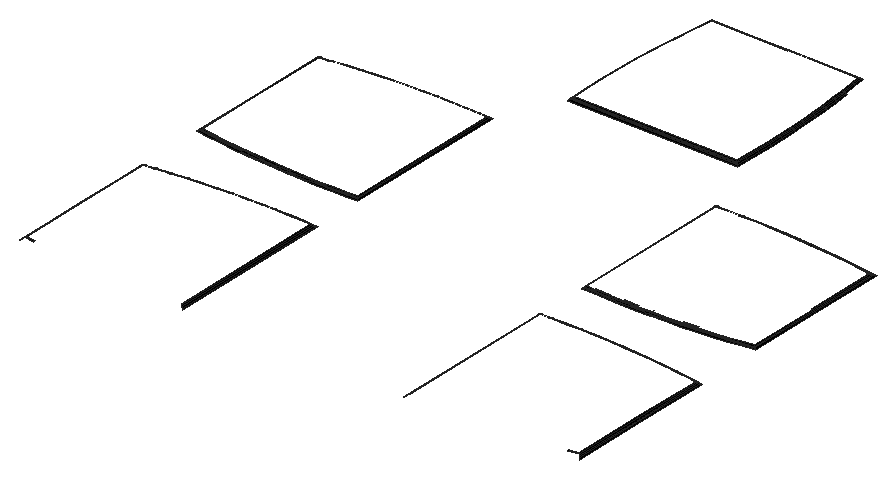
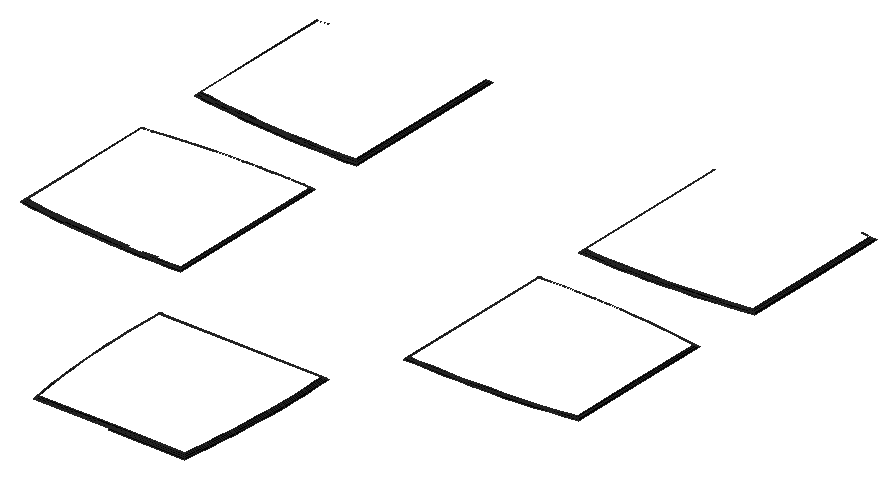
# SketchUp Ruby script. Lengths in inches.
U = 1.inch
M = Sketchup.active_model
def pt(a) = Geom::Point3d.new(a.map { |v| v * U })
def face(e, loops, mat)
  f = e.add_face(loops[0].map { |a| pt(a) })
  loops[1..].each { |l| e.add_face(l.map { |a| pt(a) }).erase! }
  f.material = f.back_material = mat if mat
  f
end
# faces: each face lists its corners as indices into pts; further lists are holes
def faces(e, pts, list, mat = nil) = list.each { |f| face(e, (f[0].is_a?(Array) ? f : [f]).map { |l| l.map { |i| pts[i] } }, mat) }
# xy, xz, yz: faces in a plane at the given z, y or x. An outline is a flat list of corners, or four numbers for a rectangle; further outlines are holes
def ring(l) = l.size == 4 ? [[l[0], l[1]], [l[2], l[1]], [l[2], l[3]], [l[0], l[3]]] : l.each_slice(2).to_a
def flat(e, list, mat, &to3) = list.each { |f| face(e, (f[0].is_a?(Array) ? f : [f]).map { |l| ring(l).map { |u, v| to3.(u, v) } }, mat) }
def xy(e, z, list, mat = nil) = flat(e, list, mat) { |x, y| [x, y, z] }
def xz(e, y, list, mat = nil) = flat(e, list, mat) { |x, z| [x, y, z] }
def yz(e, x, list, mat = nil) = flat(e, list, mat) { |y, z| [x, y, z] }
def lines(e, pts, list) = list.each { |a, b| e.add_line(pt(pts[a]), pt(pts[b])) }
# prism: a flat outline (further loops are holes) pulled along v
def prism(e, loops, v, mat = nil)
  f = face(e, loops, mat); d = Geom::Vector3d.new(v.map { |x| x * U })
  f.pushpull(f.normal.samedirection?(d) ? d.length : -d.length)
end
def box(e, o, s, mat = nil) = prism(e, [[o, [o[0] + s[0], o[1], o[2]], [o[0] + s[0], o[1] + s[1], o[2]], [o[0], o[1] + s[1], o[2]]]], [0, 0, s[2]], mat)
def at(x, y, z, deg = 0) = Geom::Transformation.translation(pt([x, y, z])) * Geom::Transformation.rotation(ORIGIN, Z_AXIS, deg.degrees)
def axes(o, x, y, z) = Geom::Transformation.new([*x, 0, *y, 0, *z, 0, *pt(o).to_a, 1])
def part(name) = M.definitions.add(name)
# library, detail: a bought-in or finely detailed component or shape, given as its bounding box
def library(name, o, s) = part(name).tap { |d| box(d.entities, o, s) }
def detail(e, o, s) = box(e.add_group.entities, o, s)
def put(e, d, t, mat = nil) = e.add_instance(d, t).tap { |i| i.material = mat if mat }
def group(e, t, mat = nil) = e.add_group.tap { |g| g.transformation = t; g.material = mat if mat }.entities
root = M.entities
M.materials.add("[Color M09]").color = [0, 0, 0]
p = [[101.197,133.183,29.641],[101.294,133.276,29.531],[101.294,113.3,29.531],[101.197,113.394,29.641],[127.526,113.394,29.641],[127.429,113.3,29.531],
  [127.429,133.276,29.531],[127.526,133.183,29.641],[81.338,114.3,29.531],[81.435,114.384,29.641],[81.435,123.288,29.641],[81.338,123.288,29.531],
  [147.289,114.384,29.641],[147.386,114.3,29.531],[147.386,123.288,29.531],[147.289,123.288,29.641],[81.435,132.192,29.641],[81.338,132.276,29.531],
  [147.386,132.276,29.531],[147.289,132.192,29.641],[82.839,132.392,29.641],[82.826,132.488,29.531],[145.898,132.488,29.531],[145.885,132.392,29.641],
  [84.527,132.603,29.641],[84.515,132.7,29.531],[144.208,132.7,29.531],[144.197,132.603,29.641],[86.218,132.787,29.641],[86.208,132.883,29.531],
  [142.515,132.883,29.531],[142.506,132.787,29.641],[87.912,132.942,29.641],[87.904,133.039,29.531],[140.82,133.039,29.531],[140.811,132.942,29.641],
  [89.609,133.07,29.641],[89.602,133.166,29.531],[139.121,133.166,29.531],[139.115,133.07,29.641],[91.307,133.169,29.641],[91.302,133.266,29.531],
  [137.421,133.266,29.531],[137.417,133.169,29.641],[93.002,133.336,29.531],[93.004,133.239,29.641],[93.01,133.24,29.641],[93.006,133.337,29.531],
  [94.706,133.379,29.531],[94.708,133.282,29.641],[98.11,133.282,29.641],[98.112,133.38,29.531],[99.814,133.337,29.531],[99.811,133.24,29.641],
  [128.91,133.337,29.531],[128.913,133.24,29.641],[130.612,133.38,29.531],[130.614,133.282,29.641],[134.018,133.379,29.531],[135.718,133.337,29.531],
  [135.714,133.24,29.641],[134.016,133.282,29.641],[135.722,133.336,29.531],[135.72,133.239,29.641],[96.409,133.393,29.531],[96.409,133.296,29.641],
  [132.315,133.393,29.531],[132.315,133.296,29.641],[104.313,167.782,29.531],[104.41,167.785,29.641],[104.467,166.399,29.641],[104.374,166.302,29.531],
  [124.256,166.399,29.641],[124.35,166.302,29.531],[124.314,167.785,29.641],[124.411,167.782,29.531],[104.27,169.484,29.531],[104.368,169.486,29.641],
  [124.356,169.486,29.641],[124.453,169.484,29.531],[104.257,171.1875,29.531],[104.354,171.187,29.641],[124.37,171.187,29.641],[124.467,171.1875,29.531],
  [104.271,172.89,29.531],[104.368,172.889,29.641],[124.356,172.889,29.641],[124.453,172.89,29.531],[104.313,174.591,29.531],[104.41,174.587,29.641],
  [124.41,174.591,29.531],[124.313,174.587,29.641],[104.411,174.592,29.641],[104.314,174.594,29.531],[104.384,176.294,29.531],[104.481,176.289,29.641],
  [124.41,174.594,29.531],[124.339,176.294,29.531],[124.242,176.289,29.641],[124.313,174.592,29.641],[104.58,177.987,29.641],[104.484,177.994,29.531],
  [124.24,177.994,29.531],[124.143,177.987,29.641],[104.708,179.684,29.641],[104.611,179.692,29.531],[124.113,179.692,29.531],[124.016,179.684,29.641],
  [104.863,181.378,29.641],[104.767,181.388,29.531],[123.957,181.388,29.531],[123.86,181.378,29.641],[105.047,183.069,29.641],[104.95,183.081,29.531],
  [123.773,183.081,29.531],[123.677,183.069,29.641],[105.258,184.757,29.641],[105.162,184.77,29.531],[105.458,186.161,29.641],[105.374,186.258,29.531],
  [114.362,186.161,29.641],[114.362,186.258,29.531],[101.087,133.077,29.739],[101.087,113.5,29.739],[127.637,113.5,29.739],[127.637,133.077,29.739],
  [81.545,114.48,29.739],[81.545,123.288,29.739],[147.178,114.48,29.739],[147.178,123.288,29.739],[81.545,132.096,29.739],[147.178,132.096,29.739],
  [82.853,132.282,29.739],[145.87,132.282,29.739],[84.54,132.493,29.739],[144.184,132.493,29.739],[86.229,132.677,29.739],[142.495,132.677,29.739],
  [87.921,132.832,29.739],[140.802,132.832,29.739],[89.616,132.959,29.739],[139.108,132.959,29.739],[91.3125,133.058,29.739],[137.411,133.058,29.739],
  [93.007,133.129,29.739],[93.014,133.129,29.739],[94.709,133.171,29.739],[98.108,133.172,29.739],[99.807,133.13,29.739],[128.917,133.13,29.739],
  [130.615,133.172,29.739],[135.709,133.129,29.739],[134.014,133.171,29.739],[135.717,133.129,29.739],[96.409,133.186,29.739],[132.315,133.186,29.739],
  [91.307,139.314,29.641],[93.004,139.243,29.641],[93.007,139.354,29.739],[91.3125,139.424,29.739],[94.708,139.2,29.641],[93.01,139.243,29.641],
  [93.014,139.353,29.739],[94.709,139.311,29.739],[96.409,139.297,29.739],[96.409,139.186,29.641],[98.108,139.31,29.739],[98.11,139.2,29.641],
  [99.807,139.353,29.739],[99.811,139.242,29.641],[101.087,139.406,29.739],[101.197,139.299,29.641],[128.917,139.353,29.739],[128.913,139.242,29.641],
  [127.526,139.299,29.641],[127.637,139.406,29.739],[130.615,139.31,29.739],[130.614,139.2,29.641],[132.315,139.297,29.739],[132.315,139.186,29.641],
  [134.014,139.311,29.739],[134.016,139.2,29.641],[135.714,139.243,29.641],[135.709,139.353,29.739],[135.717,139.354,29.739],[135.72,139.243,29.641],
  [137.417,139.314,29.641],[137.411,139.424,29.739],[89.616,139.523,29.739],[89.609,139.413,29.641],[101.087,158.983,29.739],[101.197,159.089,29.641],
  [127.526,159.089,29.641],[127.637,158.983,29.739],[139.115,139.413,29.641],[139.108,139.523,29.739],[87.921,139.65,29.739],[87.912,139.54,29.641],
  [140.811,139.54,29.641],[140.802,139.65,29.739],[86.229,139.806,29.739],[86.218,139.695,29.641],[142.506,139.695,29.641],[142.495,139.806,29.739],
  [84.54,139.989,29.739],[84.527,139.879,29.641],[144.197,139.879,29.641],[144.184,139.989,29.739],[82.853,140.2,29.739],[82.839,140.091,29.641],
  [145.885,140.091,29.641],[145.87,140.2,29.739],[81.545,140.386,29.739],[81.435,140.29,29.641],[147.289,140.29,29.641],[147.178,140.386,29.739],
  [81.545,149.194,29.739],[81.435,149.194,29.641],[147.289,149.194,29.641],[147.178,149.194,29.739],[81.545,158.002,29.739],[81.435,158.098,29.641],
  [147.289,158.098,29.641],[147.178,158.002,29.739],[82.853,158.188,29.739],[82.839,158.298,29.641],[145.885,158.298,29.641],[145.87,158.188,29.739],
  [84.54,158.399,29.739],[84.527,158.509,29.641],[144.197,158.509,29.641],[144.184,158.399,29.739],[86.229,158.583,29.739],[86.218,158.693,29.641],
  [142.506,158.693,29.641],[142.495,158.583,29.739],[87.921,158.738,29.739],[87.912,158.848,29.641],[140.811,158.848,29.641],[140.802,158.738,29.739],
  [89.616,158.865,29.739],[89.609,158.975,29.641],[139.115,158.975,29.641],[139.108,158.865,29.739],[91.3125,158.964,29.739],[91.307,159.075,29.641],
  [137.417,159.075,29.641],[137.411,158.964,29.739],[93.004,159.145,29.641],[93.007,159.035,29.739],[93.014,159.035,29.739],[93.01,159.145,29.641],
  [94.708,159.188,29.641],[94.709,159.077,29.739],[98.108,159.078,29.739],[98.11,159.188,29.641],[99.811,159.146,29.641],[99.807,159.036,29.739],
  [128.913,159.146,29.641],[128.917,159.036,29.739],[130.614,159.188,29.641],[130.615,159.078,29.739],[134.016,159.188,29.641],[135.714,159.145,29.641],
  [135.709,159.035,29.739],[134.014,159.077,29.739],[135.72,159.145,29.641],[135.717,159.035,29.739],[96.409,159.202,29.641],[96.409,159.092,29.739],
  [132.315,159.202,29.641],[132.315,159.092,29.739],[104.52,167.789,29.739],[104.573,166.509,29.739],[124.15,166.509,29.739],[124.203,167.789,29.739],
  [104.478,169.488,29.739],[124.245,169.488,29.739],[104.464,171.187,29.739],[124.259,171.187,29.739],[104.479,172.887,29.739],[124.245,172.887,29.739],
  [104.521,174.582,29.739],[124.203,174.582,29.739],[104.521,174.589,29.739],[104.592,176.284,29.739],[124.132,176.284,29.739],[124.202,174.589,29.739],
  [104.691,177.98,29.739],[124.033,177.98,29.739],[104.818,179.675,29.739],[123.906,179.675,29.739],[104.973,181.367,29.739],[123.75,181.367,29.739],
  [105.157,183.057,29.739],[123.567,183.057,29.739],[105.368,184.743,29.739],[123.465,184.757,29.641],[123.356,184.743,29.739],[105.554,186.051,29.739],
  [123.266,186.161,29.641],[123.17,186.051,29.739],[114.362,186.051,29.739],[100.964,132.959,29.82],[100.964,113.617,29.82],[127.759,113.617,29.82],
  [127.759,132.959,29.82],[81.668,114.587,29.82],[81.668,123.288,29.82],[147.056,114.587,29.82],[147.056,123.288,29.82],[81.668,131.99,29.82],
  [147.056,131.99,29.82],[82.869,132.161,29.82],[145.854,132.161,29.82],[84.554,132.372,29.82],[144.17,132.372,29.82],[86.241,132.555,29.82],
  [142.482,132.555,29.82],[87.932,132.71,29.82],[140.792,132.71,29.82],[89.624,132.837,29.82],[139.099,132.837,29.82],[91.319,132.936,29.82],
  [137.405,132.936,29.82],[93.01,133.006,29.82],[135.714,133.006,29.82],[93.019,133.007,29.82],[94.711,133.049,29.82],[96.409,133.063,29.82],
  [98.106,133.049,29.82],[99.803,133.007,29.82],[128.921,133.007,29.82],[130.617,133.049,29.82],[132.315,133.063,29.82],[134.012,133.049,29.82],
  [135.704,133.007,29.82],[93.019,139.476,29.82],[94.711,139.433,29.82],[96.409,139.419,29.82],[98.106,139.433,29.82],[99.803,139.475,29.82],
  [130.617,139.433,29.82],[128.921,139.475,29.82],[132.315,139.419,29.82],[134.012,139.433,29.82],[135.704,139.476,29.82],[91.319,139.546,29.82],
  [89.624,139.645,29.82],[93.01,139.476,29.82],[100.964,139.523,29.82],[100.964,158.865,29.82],[127.759,139.523,29.82],[127.759,158.865,29.82],
  [135.714,139.476,29.82],[137.405,139.546,29.82],[139.099,139.645,29.82],[87.932,139.772,29.82],[140.792,139.772,29.82],[86.241,139.927,29.82],
  [142.482,139.927,29.82],[84.554,140.11,29.82],[144.17,140.11,29.82],[82.869,140.322,29.82],[145.854,140.322,29.82],[81.668,140.493,29.82],
  [147.056,140.493,29.82],[81.668,149.194,29.82],[147.056,149.194,29.82],[81.668,157.896,29.82],[147.056,157.896,29.82],[82.869,158.067,29.82],
  [145.854,158.067,29.82],[84.554,158.278,29.82],[144.17,158.278,29.82],[86.241,158.461,29.82],[142.482,158.461,29.82],[87.932,158.616,29.82],
  [140.792,158.616,29.82],[89.624,158.743,29.82],[139.099,158.743,29.82],[91.319,158.842,29.82],[137.405,158.842,29.82],[93.01,158.912,29.82],
  [135.714,158.912,29.82],[93.019,158.913,29.82],[94.711,158.955,29.82],[98.106,158.955,29.82],[99.803,158.913,29.82],[128.921,158.913,29.82],
  [130.617,158.955,29.82],[135.704,158.913,29.82],[134.012,158.955,29.82],[96.409,158.969,29.82],[132.315,158.969,29.82],[104.643,167.793,29.82],
  [104.691,166.632,29.82],[124.033,166.632,29.82],[124.081,167.793,29.82],[104.601,169.49,29.82],[124.123,169.49,29.82],[104.587,171.187,29.82],
  [124.137,171.187,29.82],[104.601,172.885,29.82],[124.123,172.885,29.82],[104.643,174.577,29.82],[124.08,174.577,29.82],[104.644,174.586,29.82],
  [104.714,176.277,29.82],[124.01,176.277,29.82],[124.08,174.586,29.82],[104.813,177.972,29.82],[123.911,177.972,29.82],[104.94,179.665,29.82],
  [123.784,179.665,29.82],[105.095,181.355,29.82],[123.629,181.355,29.82],[105.278,183.042,29.82],[123.445,183.042,29.82],[105.489,184.727,29.82],
  [123.234,184.727,29.82],[105.66,185.928,29.82],[123.063,185.928,29.82],[114.362,185.928,29.82],[100.832,132.833,29.885],[100.832,113.744,29.885],
  [127.891,113.744,29.885],[127.891,132.833,29.885],[82.869,114.416,29.82],[82.887,114.546,29.885],[81.8,114.701,29.885],[145.837,114.546,29.885],
  [145.854,114.416,29.82],[146.924,114.701,29.885],[81.8,123.288,29.885],[146.924,123.288,29.885],[81.8,131.875,29.885],[146.924,131.875,29.885],
  [82.887,132.03,29.885],[145.837,132.03,29.885],[84.569,132.241,29.885],[144.155,132.241,29.885],[86.254,132.424,29.885],[142.469,132.424,29.885],
  [87.942,132.579,29.885],[140.781,132.579,29.885],[89.633,132.705,29.885],[139.091,132.705,29.885],[91.325,132.804,29.885],[137.398,132.804,29.885],
  [93.013,132.874,29.885],[99.799,132.875,29.885],[128.925,132.875,29.885],[135.71,132.874,29.885],[93.025,132.875,29.885],[94.714,132.917,29.885],
  [96.409,132.931,29.885],[98.104,132.917,29.885],[130.62,132.917,29.885],[132.315,132.931,29.885],[134.01,132.917,29.885],[135.699,132.875,29.885],
  [93.025,139.607,29.885],[94.714,139.565,29.885],[96.409,139.551,29.885],[98.104,139.565,29.885],[99.799,139.607,29.885],[130.62,139.565,29.885],
  [128.925,139.607,29.885],[132.315,139.551,29.885],[134.01,139.565,29.885],[135.699,139.607,29.885],[91.325,139.678,29.885],[89.633,139.777,29.885],
  [93.013,139.608,29.885],[100.832,139.65,29.885],[100.832,158.738,29.885],[127.891,139.65,29.885],[127.891,158.738,29.885],[135.71,139.608,29.885],
  [137.398,139.678,29.885],[139.091,139.777,29.885],[87.942,139.904,29.885],[140.781,139.904,29.885],[86.254,140.059,29.885],[142.469,140.059,29.885],
  [84.569,140.242,29.885],[144.155,140.242,29.885],[82.887,140.452,29.885],[145.837,140.452,29.885],[81.8,140.607,29.885],[146.924,140.607,29.885],
  [81.8,149.194,29.885],[146.924,149.194,29.885],[81.8,157.781,29.885],[146.924,157.781,29.885],[82.887,157.936,29.885],[145.837,157.936,29.885],
  [84.569,158.147,29.885],[144.155,158.147,29.885],[86.254,158.33,29.885],[142.469,158.33,29.885],[87.942,158.484,29.885],[140.781,158.484,29.885],
  [89.633,158.611,29.885],[139.091,158.611,29.885],[91.325,158.71,29.885],[137.398,158.71,29.885],[93.013,158.78,29.885],[99.799,158.781,29.885],
  [128.925,158.781,29.885],[135.71,158.78,29.885],[93.025,158.781,29.885],[94.714,158.823,29.885],[96.409,158.837,29.885],[98.104,158.823,29.885],
  [130.62,158.823,29.885],[132.315,158.837,29.885],[134.01,158.823,29.885],[135.699,158.781,29.885],[104.775,167.797,29.885],[104.817,166.764,29.885],
  [123.906,166.764,29.885],[123.949,167.797,29.885],[104.733,169.492,29.885],[123.991,169.492,29.885],[104.719,171.187,29.885],[124.005,171.187,29.885],
  [104.733,172.882,29.885],[123.991,172.882,29.885],[104.775,174.571,29.885],[123.948,174.571,29.885],[104.776,174.583,29.885],[104.846,176.271,29.885],
  [123.948,174.583,29.885],[123.878,176.271,29.885],[104.945,177.963,29.885],[123.779,177.963,29.885],[105.071,179.654,29.885],[123.652,179.654,29.885],
  [105.226,181.342,29.885],[123.497,181.342,29.885],[105.409,183.027,29.885],[123.314,183.027,29.885],[105.62,184.709,29.885],[123.104,184.709,29.885],
  [105.775,185.796,29.885],[122.949,185.796,29.885],[114.362,185.796,29.885],[130.622,139.704,29.933],[128.93,139.746,29.933],[134.008,139.705,29.933],
  [132.315,139.69,29.933],[135.693,139.747,29.933],[135.707,139.747,29.933],[139.081,139.916,29.933],[140.77,140.043,29.933],[146.785,157.66,29.933],
  [146.785,149.194,29.933],[145.818,157.798,29.933],[144.138,158.008,29.933],[142.455,158.191,29.933],[140.77,158.346,29.933],[139.081,158.472,29.933],
  [137.391,158.571,29.933],[135.693,158.642,29.933],[134.008,158.684,29.933],[135.707,158.641,29.933],[132.315,158.698,29.933],[130.622,158.684,29.933]]
faces(root,p,[[0,1,2,3],[4,5,6,7],[8,9,10,11],[12,13,14,15],[16,17,11,10],[18,19,15,14],[20,21,17,16],[22,23,19,18],
  [24,25,21,20],[26,27,23,22],[28,29,25,24],[30,31,27,26],[32,33,29,28],[34,35,31,30],[36,37,33,32],[38,39,35,34],
  [40,41,37,36],[42,43,39,38],[44,41,40,45],[45,46,47,44],[47,48,49,46],[50,51,52,53],[53,52,1,0],[54,55,7,6],
  [56,57,55,54],[58,59,60,61],[42,62,63,43],[63,60,59,62],[49,48,64,65],[65,64,51,50],[66,67,57,56],[58,61,67,66],
  [68,69,70,71],[72,73,71,70],[74,75,73,72],[76,77,69,68],[78,79,75,74],[80,81,77,76],[82,83,79,78],[84,85,81,80],
  [86,87,83,82],[84,88,89,85],[90,87,86,91],[92,89,88,93],[94,93,92,95],[96,97,98,99],[99,91,90,96],[94,95,100,101],
  [98,97,102,103],[101,100,104,105],[103,102,106,107],[105,104,108,109],[107,106,110,111],[109,108,112,113],[111,110,114,115],[113,112,116,117],
  [117,116,118,119],[119,118,120,121],[122,0,3,123],[124,4,7,125],[9,126,127,10],[128,12,15,129],[130,16,10,127],[19,131,129,15],
  [132,20,16,130],[23,133,131,19],[134,24,20,132],[27,135,133,23],[136,28,24,134],[31,137,135,27],[138,32,28,136],[35,139,137,31],
  [140,36,32,138],[39,141,139,35],[142,40,36,140],[43,143,141,39],[45,40,142,144],[144,145,46,45],[46,49,146,145],[147,50,53,148],
  [148,53,0,122],[55,149,125,7],[57,150,149,55],[61,60,151,152],[43,63,153,143],[153,151,60,63],[146,49,65,154],[154,65,50,147],
  [67,155,150,57],[61,152,155,67],[156,157,158,159],[160,161,162,163],[158,162,161,157],[160,163,164,165],[165,164,166,167],[167,166,168,169],
  [169,168,170,171],[172,173,174,175],[176,177,173,172],[178,179,177,176],[180,181,179,178],[182,181,180,183],[184,183,182,185],[185,186,187,184],
  [156,159,188,189],[190,191,171,170],[175,174,192,193],[187,186,194,195],[189,188,196,197],[195,194,198,199],[197,196,200,201],[199,198,202,203],
  [201,200,204,205],[203,202,206,207],[205,204,208,209],[207,206,210,211],[209,208,212,213],[211,210,214,215],[213,212,216,217],[215,214,218,219],
  [220,221,217,216],[222,223,219,218],[224,225,221,220],[226,227,223,222],[228,229,225,224],[230,231,227,226],[232,233,229,228],[234,235,231,230],
  [236,237,233,232],[238,239,235,234],[240,241,237,236],[242,243,239,238],[244,245,241,240],[246,247,243,242],[248,245,244,249],[249,250,251,248],
  [251,252,253,250],[254,255,256,257],[257,256,191,190],[258,259,193,192],[260,261,259,258],[262,263,264,265],[246,266,267,247],[267,264,263,266],
  [253,252,268,269],[269,268,255,254],[270,271,261,260],[262,265,271,270],[69,272,273,70],[274,72,70,273],[275,74,72,274],[77,276,272,69],
  [277,78,74,275],[81,278,276,77],[279,82,78,277],[85,280,278,81],[281,86,82,279],[85,89,282,280],[91,86,281,283],[284,282,89,92],
  [95,92,284,285],[99,98,286,287],[287,283,91,99],[95,285,288,100],[286,98,103,289],[100,288,290,104],[289,103,107,291],[104,290,292,108],
  [291,107,111,293],[108,292,294,112],[293,111,115,295],[112,294,296,116],[295,115,297,298],[116,296,299,118],[298,297,300,301],[118,299,302,120],
  [301,300,120,302],[303,122,123,304],[305,124,125,306],[126,307,308,127],[309,128,129,310],[311,130,127,308],[131,312,310,129],[313,132,130,311],
  [133,314,312,131],[315,134,132,313],[135,316,314,133],[317,136,134,315],[137,318,316,135],[319,138,136,317],[139,320,318,137],[321,140,138,319],
  [141,322,320,139],[323,142,140,321],[143,324,322,141],[144,142,323,325],[143,153,326,324],[325,327,145,144],[145,146,328,327],[328,146,154,329],
  [329,154,147,330],[330,147,148,331],[331,148,122,303],[149,332,306,125],[150,333,332,149],[155,334,333,150],[152,335,334,155],[152,151,336,335],
  [336,326,153,151],[163,162,337,338],[163,338,339,164],[164,339,340,166],[166,340,341,168],[342,176,172,343],[344,178,176,342],[345,180,178,344],
  [183,180,345,346],[159,347,348,188],[159,158,349,347],[337,349,158,162],[168,341,350,170],[351,190,170,350],[343,172,175,352],[352,175,193,353],
  [354,346,183,184],[184,187,355,354],[355,187,195,356],[188,348,357,196],[356,195,199,358],[196,357,359,200],[358,199,203,360],[200,359,361,204],
  [360,203,207,362],[204,361,363,208],[362,207,211,364],[208,363,365,212],[364,211,215,366],[212,365,367,216],[366,215,219,368],[369,220,216,367],
  [223,370,368,219],[371,224,220,369],[227,372,370,223],[373,228,224,371],[231,374,372,227],[375,232,228,373],[235,376,374,231],[377,236,232,375],
  [239,378,376,235],[379,240,236,377],[243,380,378,239],[381,244,240,379],[247,382,380,243],[249,244,381,383],[247,267,384,382],[383,385,250,249],
  [250,253,386,385],[387,254,257,388],[388,257,190,351],[259,389,353,193],[261,390,389,259],[265,264,391,392],[391,384,267,264],[386,253,269,393],
  [393,269,254,387],[271,394,390,261],[265,392,394,271],[272,395,396,273],[397,274,273,396],[398,275,274,397],[276,399,395,272],[400,277,275,398],
  [278,401,399,276],[402,279,277,400],[280,403,401,278],[404,281,279,402],[280,282,405,403],[283,281,404,406],[405,407,284,282],[285,284,407,408],
  [287,286,409,410],[410,406,283,287],[285,408,411,288],[409,286,289,412],[288,411,413,290],[412,289,291,414],[290,413,415,292],[414,291,293,416],
  [292,415,417,294],[416,293,295,418],[294,417,419,296],[418,295,298,420],[296,419,421,299],[420,298,301,422],[299,421,423,302],[422,301,302,423],
  [424,303,304,425],[426,305,306,427],[428,429,430,307],[431,432,309,433],[307,430,434,308],[433,309,310,435],[436,311,308,434],[312,437,435,310],
  [438,313,311,436],[314,439,437,312],[440,315,313,438],[316,441,439,314],[442,317,315,440],[318,443,441,316],[444,319,317,442],[320,445,443,318],
  [446,321,319,444],[322,447,445,320],[448,323,321,446],[324,449,447,322],[325,323,448,450],[451,331,303,424],[332,452,427,306],[324,326,453,449],
  [454,450,325,327],[327,328,455,454],[455,328,329,456],[456,329,330,457],[457,330,331,451],[333,458,452,332],[334,459,458,333],[335,460,459,334],
  [335,336,461,460],[453,461,336,326],[338,337,462,463],[338,463,464,339],[339,464,465,340],[340,465,466,341],[467,342,343,468],[469,344,342,467],
  [470,345,344,469],[346,345,470,471],[347,472,473,348],[347,349,474,472],[474,462,337,349],[341,466,475,350],[476,351,350,475],[468,343,352,477],
  [477,352,353,478],[471,479,354,346],[354,355,480,479],[480,355,356,481],[348,473,482,357],[481,356,358,483],[357,482,484,359],[483,358,360,485],
  [359,484,486,361],[485,360,362,487],[361,486,488,363],[487,362,364,489],[363,488,490,365],[489,364,366,491],[365,490,492,367],[491,366,368,493],
  [494,369,367,492],[370,495,493,368],[496,371,369,494],[372,497,495,370],[498,373,371,496],[374,499,497,372],[500,375,373,498],[376,501,499,374],
  [502,377,375,500],[378,503,501,376],[504,379,377,502],[380,505,503,378],[506,381,379,504],[382,507,505,380],[383,381,506,508],[509,388,351,476],
  [389,510,478,353],[382,384,511,507],[512,508,383,385],[385,386,513,512],[513,386,393,514],[514,393,387,515],[515,387,388,509],[390,516,510,389],
  [394,517,516,390],[392,518,517,394],[392,391,519,518],[511,519,391,384],[395,520,521,396],[522,397,396,521],[523,398,397,522],[399,524,520,395],
  [525,400,398,523],[401,526,524,399],[527,402,400,525],[403,528,526,401],[529,404,402,527],[403,405,530,528],[406,404,529,531],[532,530,405,407],
  [408,407,532,533],[531,534,410,406],[410,409,535,534],[408,533,536,411],[535,409,412,537],[411,536,538,413],[537,412,414,539],[413,538,540,415],
  [539,414,416,541],[415,540,542,417],[541,416,418,543],[417,542,544,419],[543,418,420,545],[419,544,546,421],[545,420,422,547],[421,546,548,423],
  [547,422,423,548],[549,467,468,550],[551,470,469,552],[553,554,479,471],[555,481,483,556],[495,557,558,493],[497,559,557,495],[499,560,559,497],
  [501,561,560,499],[503,562,561,501],[505,563,562,503],[507,564,563,505],[518,519,565,566],[507,511,567,564],[565,567,511,519],[517,568,569,516]],"[Color M09]")
